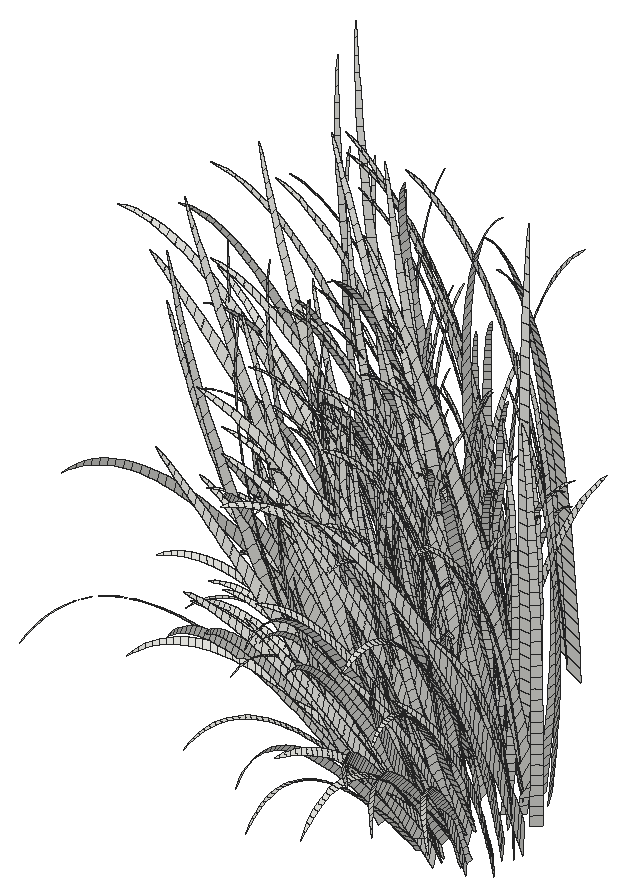
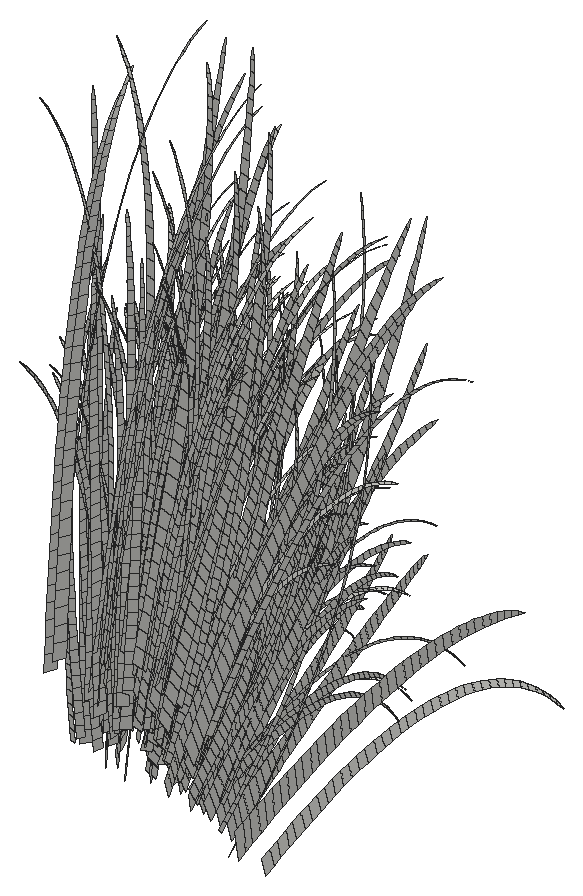
# SketchUp Ruby script. Lengths in inches.
U = 1.inch
M = Sketchup.active_model
def pt(a) = Geom::Point3d.new(a.map { |v| v * U })
def face(e, loops, mat)
  f = e.add_face(loops[0].map { |a| pt(a) })
  loops[1..].each { |l| e.add_face(l.map { |a| pt(a) }).erase! }
  f.material = f.back_material = mat if mat
  f
end
# faces: each face lists its corners as indices into pts; further lists are holes
def faces(e, pts, list, mat = nil) = list.each { |f| face(e, (f[0].is_a?(Array) ? f : [f]).map { |l| l.map { |i| pts[i] } }, mat) }
# xy, xz, yz: faces in a plane at the given z, y or x. An outline is a flat list of corners, or four numbers for a rectangle; further outlines are holes
def ring(l) = l.size == 4 ? [[l[0], l[1]], [l[2], l[1]], [l[2], l[3]], [l[0], l[3]]] : l.each_slice(2).to_a
def flat(e, list, mat, &to3) = list.each { |f| face(e, (f[0].is_a?(Array) ? f : [f]).map { |l| ring(l).map { |u, v| to3.(u, v) } }, mat) }
def xy(e, z, list, mat = nil) = flat(e, list, mat) { |x, y| [x, y, z] }
def xz(e, y, list, mat = nil) = flat(e, list, mat) { |x, z| [x, y, z] }
def yz(e, x, list, mat = nil) = flat(e, list, mat) { |y, z| [x, y, z] }
def lines(e, pts, list) = list.each { |a, b| e.add_line(pt(pts[a]), pt(pts[b])) }
# prism: a flat outline (further loops are holes) pulled along v
def prism(e, loops, v, mat = nil)
  f = face(e, loops, mat); d = Geom::Vector3d.new(v.map { |x| x * U })
  f.pushpull(f.normal.samedirection?(d) ? d.length : -d.length)
end
def box(e, o, s, mat = nil) = prism(e, [[o, [o[0] + s[0], o[1], o[2]], [o[0] + s[0], o[1] + s[1], o[2]], [o[0], o[1] + s[1], o[2]]]], [0, 0, s[2]], mat)
def at(x, y, z, deg = 0) = Geom::Transformation.translation(pt([x, y, z])) * Geom::Transformation.rotation(ORIGIN, Z_AXIS, deg.degrees)
def axes(o, x, y, z) = Geom::Transformation.new([*x, 0, *y, 0, *z, 0, *pt(o).to_a, 1])
def part(name) = M.definitions.add(name)
# library, detail: a bought-in or finely detailed component or shape, given as its bounding box
def library(name, o, s) = part(name).tap { |d| box(d.entities, o, s) }
def detail(e, o, s) = box(e.add_group.entities, o, s)
def put(e, d, t, mat = nil) = e.add_instance(d, t).tap { |i| i.material = mat if mat }
def group(e, t, mat = nil) = e.add_group.tap { |g| g.transformation = t; g.material = mat if mat }.entities
root = M.entities
c1 = part("fur_instance\#8")
p = [[-0.25,1.49,0.03],[0.25,-1.49,-0.03],[0.44,-1.47,1.51],[-0.05,1.47,1.57],[0.65,-1.44,3.05],[0.16,1.45,3.11],
  [0.86,-1.42,4.59],[0.38,1.44,4.65],[1.1,-1.39,6.13],[0.62,1.43,6.18],[1.34,-1.35,7.66],[0.875,1.42,7.72],
  [1.6,-1.32,9.19],[1.14,1.41,9.25],[1.88,-1.28,10.72],[1.43,1.41,10.78],[2.18,-1.24,12.25],[1.73,1.41,12.3],
  [2.49,-1.19,13.77],[2.05,1.41,13.82],[2.83,-1.15,15.29],[2.4,1.41,15.34],[3.18,-1.09,16.8],[2.76,1.42,16.85],
  [3.56,-1.03,18.31],[3.14,1.43,18.35],[3.96,-0.97,19.81],[3.55,1.44,19.85],[4.38,-0.91,21.3],[3.99,1.46,21.35],
  [4.84,-0.83,22.78],[4.45,1.48,22.83],[5.32,-0.76,24.26],[4.93,1.51,24.31],[5.82,-0.67,25.73],[5.45,1.54,25.77],
  [6.36,-0.59,27.18],[6,1.57,27.23],[6.93,-0.49,28.625],[6.58,1.61,28.67],[7.54,-0.39,30.05],[7.19,1.66,30.1],
  [8.18,-0.28,31.47],[7.84,1.71,31.51],[8.85,-0.16,32.86],[8.53,1.77,32.9],[9.57,-0.04,34.24],[9.25,1.83,34.27],
  [10.32,0.09,35.59],[10.02,1.9,35.625],[11.12,0.23,36.92],[10.82,1.97,36.95],[11.95,0.38,38.22],[11.67,2.06,38.25],
  [12.84,0.54,39.49],[12.57,2.14,39.52],[13.76,0.71,40.73],[13.51,2.24,40.76],[14.73,0.89,41.93],[14.49,2.34,41.95],
  [15.75,1.08,43.09],[15.52,2.45,43.11],[16.82,1.28,44.2],[16.6,2.5625,44.23],[17.93,1.5,45.27],[17.73,2.68,45.29],
  [19.08,1.73,46.28],[18.9,2.81,46.3],[20.29,1.97,47.24],[20.125,2.93,47.26],[21.53,2.22,48.13],[21.39,3.0625,48.15],
  [22.82,2.5,48.96],[22.7,3.1875,48.98],[24.14,2.8125,49.72],[24.06,3.3,49.73],[25.48,3.27,50.41]]
faces(c1.entities,p,[[0,1,2,3],[3,2,4,5],[5,4,6,7],[7,6,8,9],[9,8,10,11],[11,10,12,13],[13,12,14,15],[15,14,16,17],
  [17,16,18,19],[19,18,20,21],[21,20,22,23],[23,22,24,25],[25,24,26,27],[27,26,28,29],[29,28,30,31],[31,30,32,33],
  [33,32,34,35],[35,34,36,37],[37,36,38,39],[39,38,40,41],[41,40,42,43],[43,42,44,45],[45,44,46,47],[47,46,48,49],
  [49,48,50,51],[51,50,52,53],[53,52,54,55],[55,54,56,57],[57,56,58,59],[59,58,60,61],[61,60,62,63],[63,62,64,65],
  [65,64,66,67],[67,66,68,69],[69,68,70,71],[71,70,72,73],[73,72,74,75],[75,74,76]])
put(root,c1,axes([41.78,68.76,4.29],[-0.02161,-0.16628,-0.28389],[0.16425,-0.14433,0.32408],[-0.18224,-0.08282,0.344]))
put(root,c1,axes([41.84,66.78,2.31],[-0.07933,-0.07892,-0.44402],[0.19255,-0.17562,0.06989],[-0.14788,-0.14983,0.35337]))
put(root,c1,axes([44.52,67.33,8.31],[-0.23554,0.05296,-0.19778],[0.0198,-0.2043,-0.19606],[-0.09324,-0.11985,0.49597]))
put(root,c1,axes([44.3125,68.95,8.09],[-0.04128,-0.19919,-0.10991],[0.2038,-0.09544,0.23105],[-0.11682,-0.05581,0.46862]))
put(root,c1,axes([43.49,67.08,2.54],[0.13283,-0.0342,0.36955],[-0.05695,0.18902,0.06859],[-0.15898,-0.07225,0.3001]))
put(root,c1,axes([46.45,64.83,3.05],[-0.12873,0.10197,-0.18861],[-0.01018,-0.10343,-0.24101],[-0.11719,-0.08155,0.24232]))
put(root,c1,axes([45.73,68.05,7.22],[-0.08516,-0.14739,-0.15062],[0.16457,-0.13044,0.17116],[-0.1041,-0.04973,0.41758]))
put(root,c1,axes([46.54,64.22,3.46],[-0.15935,0.03269,-0.28558],[0.09029,-0.13292,-0.22683],[-0.09601,-0.14239,0.28508]))
put(root,c1,axes([46.54,64.65,2.75],[-0.14081,0.09765,-0.1356],[-0.01218,-0.08683,-0.27326],[-0.10036,-0.10168,0.23982]))
put(root,c1,axes([46.6875,66.09,7.04],[-0.18347,0.1171,-0.07334],[-0.07461,-0.13251,-0.22152],[-0.07812,-0.10043,0.41558]))
put(root,c1,axes([46.57,64.51,3.25],[-0.15082,0.11254,-0.07354],[-0.05779,-0.09193,-0.25822],[-0.08893,-0.09949,0.31347]))
put(root,c1,axes([46.55,66.52,6.48],[-0.149,-0.04647,-0.21352],[0.09287,-0.17245,0.02054],[-0.09229,-0.06322,0.38876]))
put(root,c1,axes([46.07,64.27,3.58],[-0.09966,0.12678,0.30336],[-0.19172,0.0268,-0.26785],[-0.07616,-0.17634,0.31506]))
put(root,c1,axes([45.32,66.42,3.76],[0.05365,-0.16969,-0.03778],[0.13986,-0.00916,0.27148],[-0.1167,-0.06341,0.32492]))
put(root,c1,axes([46.77,64.77,3.42],[-0.10552,0.13111,0.03774],[-0.1075,-0.03434,-0.24755],[-0.08294,-0.09279,0.29236]))
put(root,c1,axes([47.33,64.85,6.95],[-0.23362,0.09843,0.07428],[-0.08627,-0.11761,-0.36241],[-0.04076,-0.18596,0.42692]))
put(root,c1,axes([46.52,65.09,3.13],[-0.05906,0.14196,0.06951],[-0.12604,0.00717,-0.23329],[-0.09379,-0.07416,0.28621]))
put(root,c1,axes([45.22,65.05,2.3],[0.08197,-0.14846,-0.17255],[0.1435,-0.03613,0.3122],[-0.11735,-0.1189,0.28043]))
put(root,c1,axes([47.35,67.41,9.96],[-0.2227,-0.02851,-0.13015],[0.07795,-0.20389,-0.10631],[-0.04666,-0.10194,0.51151]))
put(root,c1,axes([46.74,65.87,3.48],[-0.05395,-0.10392,-0.15053],[0.10796,-0.10426,0.17042],[-0.10255,-0.03484,0.272]))
put(root,c1,axes([47.33,64.13,4.18],[-0.17727,0.00029,-0.20455],[0.08516,-0.1353,-0.21935],[-0.05731,-0.14134,0.34686]))
put(root,c1,axes([47.08,64.61,4.05],[-0.10062,-0.049,-0.26041],[0.12035,-0.13237,-0.01381],[-0.08638,-0.09663,0.30447]))
put(root,c1,axes([47.39,66.22,4.66],[-0.12457,-0.03797,-0.15408],[0.05979,-0.14532,0.07008],[-0.07901,-0.02356,0.31353]))
put(root,c1,axes([47.03,64.01,4.63],[-0.15374,0.14658,0.25603],[-0.19784,-0.04817,-0.27014],[-0.04101,-0.18709,0.42951]))
put(root,c1,axes([45.42,65.41,2.3],[0.13307,-0.06357,0.27984],[-0.03809,0.14212,0.17121],[-0.12562,-0.08741,0.25976]))
put(root,c1,axes([47.3,64.3,2.92],[-0.0986,0.1202,0.03133],[-0.09749,-0.03341,-0.22837],[-0.07635,-0.08541,0.26912]))
put(root,c1,axes([47.09,64.0625,2.52],[-0.08725,-0.02366,-0.29756],[0.12591,-0.11202,-0.06714],[-0.0803,-0.1191,0.23844]))
put(root,c1,axes([47.62,64.14,3.49],[-0.15103,0.03829,-0.1475],[0.02836,-0.11444,-0.19385],[-0.06472,-0.10394,0.28282]))
put(root,c1,axes([44.92,65.9,4.11],[0.17403,-0.06722,0.24815],[-0.01797,0.16553,0.179],[-0.11789,-0.09322,0.35975]))
put(root,c1,axes([46.59,63.5625,2.5],[-0.07738,0.12181,0.42116],[-0.24475,0.02807,-0.19007],[-0.04925,-0.2161,0.35893]))
put(root,c1,axes([47.8,63.58,3.5],[-0.19758,0.0885,0.1271],[-0.09447,-0.05952,-0.37318],[-0.04202,-0.18438,0.30623]))
put(root,c1,axes([46.29,65.45,3.97],[0.04667,0.10587,0.22641],[-0.14224,0.11026,-0.13144],[-0.10087,-0.07976,0.30781]))
put(root,c1,axes([47.18,65,6.72],[-0.12023,0.16893,0.15811],[-0.19192,-0.04724,-0.20175],[-0.05017,-0.13536,0.45159]))
put(root,c1,axes([47.44,64.82,5.0625],[-0.1513,-0.02821,-0.17374],[0.08683,-0.1419,-0.10144],[-0.05423,-0.09755,0.35603]))
put(root,c1,axes([47.56,64.62,3.98],[-0.07947,0.12548,0.07397],[-0.11521,-0.01055,-0.22059],[-0.07706,-0.08621,0.27164]))
put(root,c1,axes([47.27,66.85,4.41],[-0.06439,-0.12354,-0.04587],[0.12333,-0.08786,0.16125],[-0.07712,-0.0102,0.31415]))
put(root,c1,axes([46.72,65.11,3.03],[0.02731,-0.14018,-0.06519],[0.12315,-0.02871,0.2214],[-0.09827,-0.0534,0.27359]))
put(root,c1,axes([46.11,64.66,2.43],[0.09631,-0.13966,-0.10726],[0.11682,-0.00954,0.30869],[-0.10751,-0.10893,0.25692]))
put(root,c1,axes([48.04,64.74,5.63],[-0.18173,0.02045,-0.09763],[0.0261,-0.14072,-0.18343],[-0.04068,-0.10974,0.36609]))
put(root,c1,axes([46.52,65.89,3.82],[0.06905,-0.15041,0.07394],[0.1069,0.0384,0.22809],[-0.10814,-0.03674,0.28683]))
put(root,c1,axes([46.49,66.28,5.39],[0.02994,-0.16585,-0.05499],[0.16129,-0.01842,0.19273],[-0.08623,-0.05907,0.36324]))
put(root,c1,axes([48.125,63.5,3.07],[-0.18497,0.04944,-0.02341],[-0.00878,-0.07542,-0.33252],[-0.03553,-0.1559,0.25894]))
put(root,c1,axes([47.84,65.75,5.99],[-0.14413,-0.05167,-0.11933],[0.08701,-0.14734,-0.01287],[-0.04763,-0.0596,0.37283]))
put(root,c1,axes([47.56,63.85,2.69],[-0.04193,0.09854,0.23039],[-0.14173,0.04993,-0.18317],[-0.07748,-0.11492,0.23007]))
put(root,c1,axes([47.32,66.04,4.73],[-0.02354,-0.13666,-0.06934],[0.13862,-0.06024,0.1585],[-0.07899,-0.03774,0.31687]))
put(root,c1,axes([48.28,63.625,3.125],[-0.15528,0.03655,-0.09389],[0.01601,-0.10098,-0.21878],[-0.04549,-0.11219,0.27533]))
put(root,c1,axes([48.32,64.46,4.68],[-0.15238,0.03287,-0.097],[0.00948,-0.12228,-0.14695],[-0.04746,-0.08538,0.3116]))
put(root,c1,axes([47.56,65.7,5.13],[-0.02967,-0.13006,-0.11002],[0.14258,-0.07093,0.13984],[-0.07655,-0.05244,0.32247]))
put(root,c1,axes([46.44,65.01,3.49],[0.10962,-0.14134,0.02858],[0.09848,0.05163,0.25611],[-0.09929,-0.07851,0.30299]))
put(root,c1,axes([47.93,65.02,5.84],[-0.07622,0.14548,0.11566],[-0.15943,-0.01772,-0.1678],[-0.05494,-0.09882,0.36066]))
put(root,c1,axes([48.65,65.69,8.6],[-0.23536,0.00031,-0.04255],[0.03502,-0.16941,-0.26023],[-0.00865,-0.15175,0.46324]))
put(root,c1,axes([47.03,63.92,2.59],[0.07176,0.04443,0.32956],[-0.1495,0.11571,0.02095],[-0.08693,-0.12893,0.25813]))
put(root,c1,axes([48.18,67.92,9.34],[-0.16552,-0.11118,-0.05649],[0.14207,-0.16762,-0.00154],[-0.02412,-0.05905,0.48802]))
put(root,c1,axes([48.14,63.68,3.9375],[-0.1192,0.12425,0.22535],[-0.17166,-0.03356,-0.21354],[-0.0342,-0.15606,0.35826]))
put(root,c1,axes([47.85,65.45,5.16],[-0.02927,-0.12714,-0.10789],[0.13946,-0.06963,0.13664],[-0.0749,-0.05131,0.31553]))
put(root,c1,axes([46.1,64.84,4.72],[0.13498,-0.15634,-0.12045],[0.15269,0.03421,0.29976],[-0.08583,-0.13785,0.37509]))
put(root,c1,axes([47.34,66.07,8.47],[-0.00008,0.17023,0.2439],[-0.22913,0.05018,-0.08813],[-0.05076,-0.13695,0.4569]))
put(root,c1,axes([46.17,66.21,6.04],[0.15632,-0.13539,0.07566],[0.09629,0.11232,0.20743],[-0.0859,-0.08088,0.3964]))
put(root,c1,axes([46.0625,63.875,2.7],[0.17581,0.00429,0.35889],[-0.15371,0.13999,0.25001],[-0.08231,-0.1906,0.34052]))
put(root,c1,axes([47.25,65.44,6.82],[0.05112,0.14176,0.22694],[-0.19757,0.09246,-0.06236],[-0.06344,-0.11412,0.4165]))
put(root,c1,axes([47.59,65.46,5.51],[0.0229,-0.1484,-0.09458],[0.15576,-0.02704,0.16403],[-0.07366,-0.06935,0.33993]))
put(root,c1,axes([47.875,67.02,8.52],[-0.04613,-0.168,-0.12838],[0.20048,-0.07761,0.07112],[-0.05022,-0.08162,0.45074]))
put(root,c1,axes([47.39,66.9375,7.59],[0.01336,-0.18156,-0.05149],[0.1916,-0.02315,0.12623],[-0.05991,-0.05859,0.42926]))
put(root,c1,axes([46.94,65.12,3.85],[0.13306,-0.03251,0.2141],[-0.03468,0.1366,0.1095],[-0.09265,-0.07326,0.28274]))
put(root,c1,axes([48.44,65.3,7.09],[-0.14651,-0.09517,-0.11625],[0.13838,-0.13795,-0.08263],[-0.01824,-0.0963,0.42995]))
put(root,c1,axes([49.16,66.82,9.55],[-0.22374,-0.02944,-0.01516],[0.05551,-0.18692,-0.16154],[0.00543,-0.11272,0.49003]))
put(root,c1,axes([48.06,63.75,3.63],[-0.00857,-0.10681,-0.26092],[0.17656,-0.05814,0.06779],[-0.05152,-0.12704,0.31177]))
put(root,c1,axes([46.96,64.66,4.28],[0.14194,0.01295,0.23971],[-0.09799,0.13483,0.13149],[-0.07264,-0.11667,0.31745]))
put(root,c1,axes([47.82,64.1875,3.83],[0.04246,-0.11664,-0.17724],[0.14637,-0.02684,0.16417],[-0.06419,-0.10309,0.2805]))
put(root,c1,axes([48.97,66.82,7.8],[-0.13872,-0.10688,-0.05008],[0.13478,-0.14007,-0.01499],[-0.01621,-0.05768,0.43132]))
put(root,c1,axes([48.61,67.18,7.55],[-0.09202,-0.14419,-0.02135],[0.16494,-0.10399,0.03603],[-0.02333,-0.03794,0.42396]))
put(root,c1,axes([47.79,66.01,5.16],[0.09225,-0.12894,0.11038],[0.10291,0.0771,0.12838],[-0.07903,-0.02356,0.31361]))
put(root,c1,axes([47.93,63.42,2.29],[0.04168,-0.09258,-0.28201],[0.16554,-0.04371,0.15063],[-0.06017,-0.13932,0.24891]))
put(root,c1,axes([47.09,64.72,4.5],[0.15549,-0.01208,0.20833],[-0.06905,0.13306,0.17126],[-0.07165,-0.11508,0.31313]))
put(root,c1,axes([49.47,65.93,7.63],[-0.18618,-0.03996,-0.02577],[0.06509,-0.15689,-0.1364],[0.00464,-0.09644,0.41925]))
put(root,c1,axes([49.48,65.55,6.21],[-0.15853,0.06077,0.01255],[-0.05151,-0.13731,-0.04414],[-0.00488,-0.05314,0.37046]))
put(root,c1,axes([49.9,64.09,5.82],[-0.25079,-0.01126,0.01167],[0.02691,-0.14432,-0.37072],[0.02191,-0.19373,0.42855]))
put(root,c1,axes([49.36,63.75,4.3125],[-0.15193,-0.01941,-0.09588],[0.0644,-0.09304,-0.22233],[-0.00624,-0.12588,0.27933]))
put(root,c1,axes([49.66,62.98,2.04],[-0.16406,0.03446,0.0684],[-0.03839,-0.06194,-0.29017],[-0.00638,-0.14462,0.2315]))
put(root,c1,axes([46.76,63.98,2.88],[0.18766,-0.05407,0.15304],[-0.0375,0.10124,0.3241],[-0.06745,-0.15619,0.27904]))
put(root,c1,axes([48.46,65.78,9],[-0.04308,0.17847,0.273],[-0.24701,-0.00413,-0.05166],[-0.00912,-0.15991,0.48813]))
put(root,c1,axes([47.83,64.11,4.75],[0.03417,-0.12525,-0.29157],[0.20378,-0.0224,0.09589],[-0.03382,-0.15429,0.3542]))
put(root,c1,axes([48.12,64.54,6.09],[0.00591,-0.15376,-0.2335],[0.21361,-0.03099,0.04882],[-0.02765,-0.13326,0.41924]))
put(root,c1,axes([48.92,64.44,6.04],[-0.06192,0.14505,0.21697],[-0.19671,-0.02273,-0.07174],[-0.0075,-0.13152,0.40147]))
put(root,c1,axes([50.16,63.75,4.72],[-0.22603,-0.01056,0.00948],[0.02497,-0.13008,-0.33426],[0.01976,-0.17466,0.38636]))
put(root,c1,axes([48.68,65.36,7.52],[0.0038,0.14954,0.23139],[-0.20994,0.03733,-0.03743],[-0.02717,-0.13094,0.41195]))
put(root,c1,axes([48.78,65.625,5.72],[-0.04654,-0.13259,-0.03011],[0.14978,-0.05997,0.02545],[-0.01873,-0.03986,0.3514]))
put(root,c1,axes([48.82,63.08,2.03],[-0.02123,-0.06781,-0.31584],[0.17417,-0.05199,-0.00113],[-0.03366,-0.14772,0.24534]))
put(root,c1,axes([49.7,64.51,6.78],[-0.18897,-0.07724,-0.16578],[0.14014,-0.11074,-0.30364],[0.02044,-0.18069,0.39971]))
put(root,c1,axes([48.85,65.26,7.03],[-0.0211,0.16438,0.13367],[-0.19675,0.00758,-0.04177],[-0.01791,-0.09455,0.42215]))
put(root,c1,axes([49.51,66.02,7.33],[-0.1296,-0.11177,-0.03307],[0.13714,-0.12794,-0.0397],[-0.00189,-0.06022,0.41924]))
put(root,c1,axes([48.35,63.68,3.39],[0.0606,-0.10906,-0.18612],[0.14677,-0.00638,0.15494],[-0.04628,-0.11412,0.28007]))
put(root,c1,axes([49.9375,65.31,7.9375],[-0.15736,0.12863,0.21317],[-0.17096,-0.10355,-0.14422],[0.01307,-0.14881,0.45294]))
put(root,c1,axes([49.875,64.49,5.75],[-0.16225,-0.04777,-0.05886],[0.07812,-0.11873,-0.19059],[0.01013,-0.11533,0.35104]))
put(root,c1,axes([49.71,65.42,6.76],[-0.13495,-0.09194,-0.07228],[0.12419,-0.11921,-0.10694],[0.00432,-0.08968,0.38985]))
put(root,c1,axes([48.85,66.05,7.53],[-0.00432,-0.15952,-0.128],[0.19173,-0.03266,0.04648],[-0.02798,-0.08806,0.41192]))
put(root,c1,axes([48.375,63.94,4.2],[0.10535,0.0488,0.23666],[-0.12967,0.10407,0.09442],[-0.04869,-0.12008,0.29468]))
put(root,c1,axes([48.85,66.96,6.97],[-0.00822,-0.16722,0.01164],[0.17876,-0.02595,0.03382],[-0.01925,-0.0303,0.40131]))
put(root,c1,axes([49.99,64.4,5.2],[-0.14242,0.06423,0.07833],[-0.06984,-0.11466,-0.07925],[0.01251,-0.07634,0.33832]))
put(root,c1,axes([50.04,64.98,6.57],[-0.1422,0.11091,0.11586],[-0.12628,-0.11191,-0.06649],[0.015,-0.09153,0.40561]))
put(root,c1,axes([50.3,67.46,8.9],[-0.17633,-0.09809,0.01724],[0.1199,-0.16919,-0.04915],[0.01352,-0.05835,0.47546]))
put(root,c1,axes([50.07,63.61,4.08],[-0.13701,0.06738,0.19305],[-0.11347,-0.07671,-0.17654],[0.01546,-0.13663,0.30225]))
put(root,c1,axes([50.05,65.19,6.03],[-0.14765,0.06695,0.09599],[-0.07527,-0.12279,-0.06548],[0.02169,-0.07701,0.35566]))
put(root,c1,axes([50.42,67.52,9.97],[-0.22223,-0.05187,0.06437],[0.06185,-0.19269,-0.14793],[0.04097,-0.1013,0.49904]))
put(root,c1,axes([48.05,66.37,6.47],[0.1666,-0.05285,0.10887],[0.0248,0.15525,0.04679],[-0.05548,-0.04238,0.37888]))
put(root,c1,axes([49.94,63.07,2.46],[-0.13424,-0.03889,-0.12787],[0.08866,-0.05443,-0.25596],[0.01839,-0.13945,0.22254]))
put(root,c1,axes([49.15,64.55,5.62],[0.0286,0.11518,0.18982],[-0.16763,0.04809,-0.0018],[-0.022,-0.10604,0.33361]))
put(root,c1,axes([48.57,64.7,5.24],[0.09089,0.09523,0.11248],[-0.12952,0.09997,0.00707],[-0.03129,-0.06837,0.34303]))
put(root,c1,axes([49.31,64.97,5.66],[0.0055,0.12915,0.11043],[-0.15799,0.02454,-0.01796],[-0.01431,-0.07554,0.33727]))
put(root,c1,axes([47.59,66.85,8.375],[0.2061,-0.01344,0.1131],[-0.02793,0.18662,0.09605],[-0.05077,-0.08252,0.4557]))
put(root,c1,axes([49.52,63.37,3.39],[-0.02267,0.09523,0.24051],[-0.16406,0.00552,-0.03477],[-0.00627,-0.12634,0.28034]))
put(root,c1,axes([48.4,65.7,6.31],[0.13539,0.06511,0.11886],[-0.10233,0.13809,0.02305],[-0.04143,-0.06734,0.37184]))
put(root,c1,axes([50.24,66.6,7.25],[-0.12883,-0.11449,0.01319],[0.1336,-0.12723,-0.04151],[0.01291,-0.04776,0.41418]))
put(root,c1,axes([48.67,66.85,10.16],[0.02992,-0.20268,-0.17218],[0.24479,0.00013,0.02509],[-0.00825,-0.12029,0.52424]))
put(root,c1,axes([50.33,68.1,10.78],[-0.1863,-0.12854,0.00057],[0.15019,-0.16226,-0.16735],[0.0425,-0.10509,0.5177]))
put(root,c1,axes([49.84,66.31,6.62],[-0.07961,-0.13689,0.01423],[0.15313,-0.0843,-0.034],[0.01219,-0.0383,0.38556]))
put(root,c1,axes([49.83,66.73,7.03],[-0.07772,-0.14595,0.01956],[0.16231,-0.0838,-0.0308],[0.01178,-0.03674,0.40206]))
put(root,c1,axes([49.89,66.22,6.24],[-0.07124,-0.13476,0.02236],[0.14958,-0.07747,-0.02272],[0.00941,-0.03103,0.37011]))
put(root,c1,axes([49.61,63.66,4.18],[0.01737,0.09262,0.24572],[-0.16736,0.02852,0.02395],[-0.00637,-0.12835,0.28481]))
put(root,c1,axes([47.98,67.91,10.81],[0.18706,-0.15692,-0.05371],[0.1539,0.13296,0.16341],[-0.03534,-0.11123,0.5203]))
put(root,c1,axes([48.73,64.9375,5.4375],[0.13738,0.0414,0.0972],[-0.07592,0.13055,0.05523],[-0.03104,-0.06782,0.34028]))
put(root,c1,axes([50.12,64.96,6.6],[-0.07914,0.12591,0.21103],[-0.17333,-0.05924,-0.02394],[0.02804,-0.12033,0.37519]))
put(root,c1,axes([50.22,64.61,5.97],[-0.10701,-0.11213,-0.12442],[0.15233,-0.07687,-0.16606],[0.02739,-0.11756,0.36656]))
put(root,c1,axes([50.87,64.56,5.34],[-0.16995,0.00239,0.1052],[-0.0155,-0.13112,-0.16118],[0.04006,-0.1041,0.34197]))
put(root,c1,axes([48.71,63.27,2.98],[0.11054,0.06076,0.32124],[-0.18174,0.06569,0.1961],[-0.00805,-0.18258,0.29226]))
put(root,c1,axes([49.21,66.46,8.56],[0.04164,-0.17352,-0.14577],[0.20763,0.01338,0.03275],[-0.00709,-0.10329,0.45016]))
put(root,c1,axes([49.16,63.36,3.25],[0.07036,0.07691,0.22077],[-0.15002,0.05652,0.10186],[-0.00627,-0.1264,0.28049]))
put(root,c1,axes([48.73,65.46,6.65],[0.15043,0.06237,0.10618],[-0.10193,0.14112,0.07332],[-0.02651,-0.08344,0.39031]))
put(root,c1,axes([48.8125,64.57,5.39],[0.1599,-0.01285,0.09328],[-0.0299,0.12534,0.15874],[-0.03604,-0.09723,0.32437]))
put(root,c1,axes([51.14,63.47,3.49],[-0.19796,-0.00213,0.19119],[-0.0584,-0.09827,-0.32515],[0.05556,-0.17894,0.29438]))
put(root,c1,axes([49.65,64.5,5.97],[-0.00485,-0.13574,-0.20923],[0.19174,-0.01245,-0.03687],[0.01079,-0.12284,0.3739]))
put(root,c1,axes([48.62,64.14,4.84],[0.16477,0.01322,0.09468],[-0.05646,0.12716,0.16983],[-0.02254,-0.10862,0.34171]))
put(root,c1,axes([51.28,66.57,7.14],[-0.18521,-0.02955,0.11381],[0.03239,-0.17376,-0.06029],[0.05035,-0.05919,0.41626]))
put(root,c1,axes([51.02,64.2,4.41],[-0.14955,-0.02951,0.08847],[0.01953,-0.12021,-0.14832],[0.04773,-0.08667,0.30915]))
put(root,c1,axes([49,63.6,3.82],[0.16669,-0.01734,0.08094],[-0.02966,0.10281,0.23812],[-0.02771,-0.12642,0.29024]))
put(root,c1,axes([49.2,63.39,3.51],[0.12347,0.06755,0.21237],[-0.14396,0.08585,0.17984],[-0.00718,-0.14468,0.32104]))
put(root,c1,axes([51.18,65.25,7.42],[-0.16708,-0.12567,-0.06302],[0.15179,-0.11958,-0.24667],[0.05298,-0.1377,0.45233]))
put(root,c1,axes([49.3,67.21,6.92],[0.10751,-0.14401,0.02773],[0.14274,0.0886,-0.01156],[-0.00773,-0.0245,0.39927]))
put(root,c1,axes([50.39,63.22,2.98],[-0.04322,-0.08103,-0.33227],[0.19342,-0.01502,-0.11763],[0.02265,-0.17179,0.27415]))
put(root,c1,axes([50.66,66.19,5.78],[-0.08777,-0.12311,0.07978],[0.13105,-0.09185,-0.0647],[0.04014,-0.02395,0.34954]))
put(root,c1,axes([51.1875,64.67,6.28],[-0.14817,-0.12463,-0.07303],[0.15181,-0.10509,-0.22784],[0.04979,-0.1294,0.42509]))
put(root,c1,axes([49.47,64.26,5.16],[0.12885,0.05972,0.11755],[-0.10424,0.10176,0.1411],[-0.00603,-0.1057,0.32265]))
put(root,c1,axes([51.13,63.19,2.1],[-0.14554,-0.04613,0.08103],[0.01279,-0.07284,-0.26823],[0.06295,-0.12513,0.21981]))
put(root,c1,axes([51.38,64.25,5.13],[-0.14966,0.06135,0.2769],[-0.12806,-0.11932,-0.12286],[0.06613,-0.14624,0.35295]))
put(root,c1,axes([51.13,63.18,2.18],[-0.08929,0.05587,0.30832],[-0.15159,-0.06244,-0.09121],[0.04736,-0.15254,0.25094]))
put(root,c1,axes([49.3,65.71,6.21],[0.16373,-0.03857,0.00921],[0.02397,0.14494,0.04432],[-0.01107,-0.05099,0.36849]))
put(root,c1,axes([50.56,65.56,5.93],[-0.04201,-0.14205,-0.02716],[0.15521,-0.03808,-0.10788],[0.03986,-0.0584,0.35377]))
put(root,c1,axes([49.49,63.04,2.3],[0.15269,-0.07243,-0.24019],[0.13551,0.04613,0.26977],[-0.00773,-0.17522,0.28049]))
put(root,c1,axes([49.54,64.98,5.84],[0.14874,-0.07113,-0.04632],[0.06911,0.1145,0.10604],[-0.00549,-0.08,0.34865]))
put(root,c1,axes([51.38,65.57,5.34],[-0.14662,-0.03521,0.15792],[0.02351,-0.14317,-0.07806],[0.07228,-0.05609,0.32502]))
put(root,c1,axes([49.42,66.05,6.65],[0.16142,-0.07143,-0.01571],[0.0631,0.13884,0.04506],[-0.00507,-0.05525,0.3852]))
put(root,c1,axes([49.45,67.26,8.02],[0.12208,-0.15013,-0.02869],[0.15272,0.10311,-0.03034],[0.01381,-0.04339,0.43679]))
put(root,c1,axes([51.625,64.5625,6.29],[-0.10088,0.13062,0.3695],[-0.228,-0.07812,-0.04804],[0.0527,-0.18996,0.43195]))
put(root,c1,axes([49.73,63,2.23],[0.1143,0.07759,0.29786],[-0.18253,0.04472,0.24081],[0.02462,-0.18668,0.29791]))
put(root,c1,axes([49.9,65.15,6.76],[0.10618,-0.13596,-0.12929],[0.15853,0.08066,0.0353],[0.01505,-0.09183,0.40695]))
put(root,c1,axes([51.01,64.25,5.47],[-0.04153,-0.12718,-0.27595],[0.20481,-0.00989,-0.14624],[0.04417,-0.15922,0.36205]))
put(root,c1,axes([49.59,63.21,3.07],[0.19045,-0.03751,-0.06848],[0.03839,0.07261,0.33686],[-0.00736,-0.16676,0.26694]))
put(root,c1,axes([50.17,65.09,6.18],[0.0987,0.11897,0.05521],[-0.14378,0.08662,0.10909],[0.02282,-0.08103,0.37425]))
put(root,c1,axes([50.14,66.72,6.34],[0.11708,-0.12342,-0.00631],[0.12225,0.10057,-0.03033],[0.0076,-0.02912,0.37804]))
put(root,c1,axes([50.12,63.2,2.97],[0.10158,-0.06914,-0.32205],[0.1701,0.0448,0.14301],[0.02265,-0.17174,0.27406]))
put(root,c1,axes([51.04,63.58,3.59],[0.00165,-0.10984,-0.26082],[0.18149,0.01453,-0.07449],[0.03836,-0.13829,0.31445]))
put(root,c1,axes([52.35,65.85,7.3],[-0.1604,-0.13739,-0.02167],[0.15059,-0.11716,-0.25101],[0.06963,-0.12643,0.45099]))
put(root,c1,axes([53.03,64.98,5.97],[-0.21667,0.03837,0.29524],[-0.10928,-0.16078,-0.2283],[0.08148,-0.18018,0.43484]))
put(root,c1,axes([50.07,63.9,4.52],[0.15315,-0.04031,-0.07636],[0.04669,0.1064,0.16007],[0.009,-0.10254,0.31211]))
put(root,c1,axes([52.5,64.41,4.1875],[-0.18644,-0.03104,0.19118],[-0.0143,-0.14214,-0.22961],[0.08573,-0.13206,0.3504]))
put(root,c1,axes([50.83,65.08,5.99],[0.0438,-0.14683,-0.11127],[0.16937,0.03664,-0.05087],[0.03107,-0.07683,0.37846]))
put(root,c1,axes([52.51,67.99,10.49],[-0.20857,-0.13075,0.08955],[0.12369,-0.16885,-0.26752],[0.09431,-0.12712,0.50956]))
put(root,c1,axes([50.35,65.82,5.9],[0.13914,-0.08385,-0.03496],[0.08075,0.12335,-0.00894],[0.01158,-0.03859,0.35924]))
put(root,c1,axes([52.07,63.78,2.13],[-0.12758,-0.07753,0.0557],[0.04435,-0.06394,-0.27127],[0.08127,-0.11212,0.2187]))
put(root,c1,axes([52.35,64.0625,2.84],[-0.14977,-0.06071,0.14936],[0.00439,-0.0935,-0.26844],[0.09015,-0.12438,0.2426]))
put(root,c1,axes([51.72,64.36,3.93],[-0.08522,-0.11751,-0.02593],[0.11177,-0.04315,-0.23298],[0.08081,-0.09116,0.27707]))
put(root,c1,axes([50.51,63.84,4.31],[0.12624,-0.07118,-0.14847],[0.09892,0.09301,0.09957],[0.0236,-0.10128,0.3158]))
put(root,c1,axes([50.33,65.81,6.67],[0.11075,-0.11944,-0.11937],[0.13443,0.0987,-0.0216],[0.03784,-0.07056,0.38011]))
put(root,c1,axes([49.5625,66.85,10.4375],[0.24074,-0.08114,-0.0797],[0.07823,0.19128,0.15934],[0.00596,-0.12377,0.53808]))
put(root,c1,axes([53.36,64.16,3.67],[-0.23798,-0.07441,0.13592],[0.01899,-0.11962,-0.43721],[0.10286,-0.20447,0.35918]))
put(root,c1,axes([51.99,64.73,4.11],[-0.09743,0.06774,0.23139],[-0.09599,-0.11967,0.05358],[0.09249,-0.07723,0.28321]))
put(root,c1,axes([51.64,64.89,5.91],[-0.02184,-0.15888,-0.15748],[0.19236,-0.00034,-0.15603],[0.06127,-0.11125,0.39683]))
put(root,c1,axes([50.43,65.52,5.86],[0.15222,0.03642,-0.07852],[-0.03946,0.13914,0.07531],[0.03898,-0.05711,0.34597]))
put(root,c1,axes([52.34,65.35,3.95],[-0.11286,0.04976,0.22948],[-0.06771,-0.13658,0.05175],[0.0986,-0.05954,0.28318]))
put(root,c1,axes([51.05,66.85,6.82],[0.07494,-0.15978,-0.03962],[0.16264,0.06715,-0.11216],[0.04856,-0.037,0.39794]))
put(root,c1,axes([52.39,65.16,5.16],[-0.12334,-0.12969,0.01714],[0.11431,-0.07492,-0.27994],[0.09668,-0.10907,0.33149]))
put(root,c1,axes([50.88,63.32,2.99],[0.09702,-0.05494,-0.31246],[0.152,0.06601,0.10474],[0.04854,-0.15634,0.25719]))
put(root,c1,axes([52.02,68.49,10.01],[-0.02329,-0.21903,-0.03429],[0.23378,-0.02287,-0.15724],[0.06291,-0.07396,0.52011]))
put(root,c1,axes([50.81,66.1,5.52],[0.13682,-0.07692,-0.07129],[0.07213,0.1295,-0.07116],[0.03936,-0.02349,0.34277]))
put(root,c1,axes([50.36,63.61,4.39],[0.22137,0.04305,0.07377],[-0.08148,0.12835,0.33894],[0.02049,-0.18118,0.40078]))
put(root,c1,axes([50.76,63.89,4.47],[0.16263,0.05278,0.0273],[-0.0671,0.09353,0.2615],[0.03718,-0.13404,0.3048]))
put(root,c1,axes([50.64,66.0625,6.28],[0.1463,-0.07615,-0.10409],[0.07711,0.13848,-0.04067],[0.04559,-0.04329,0.3674]))
put(root,c1,axes([52.79,66.03,4.71],[-0.14023,0.01888,0.26296],[-0.04453,-0.1614,-0.00292],[0.11023,-0.06656,0.31656]))
put(root,c1,axes([52.66,64.38,2.89],[-0.13012,-0.10057,0.10963],[0.04873,-0.08061,-0.28847],[0.10836,-0.10823,0.24566]))
put(root,c1,axes([51.23,65.97,5.6],[0.10839,-0.11453,-0.08174],[0.11795,0.10157,-0.07097],[0.04416,-0.04194,0.35588]))
put(root,c1,axes([51.03,65.1,7.5],[0.14666,-0.13638,-0.25039],[0.18844,0.10867,0.09026],[0.03514,-0.1508,0.47019]))
put(root,c1,axes([53.0625,66.26,4.54],[-0.14894,-0.04461,0.24591],[0.01234,-0.15892,-0.10432],[0.11196,-0.06761,0.32156]))
put(root,c1,axes([52.61,68.4,9.23],[-0.02212,-0.21398,-0.03391],[0.22838,-0.02174,-0.15347],[0.06144,-0.07223,0.50797]))
put(root,c1,axes([50.58,66.9,9.57],[0.23315,0.01342,-0.06471],[-0.02237,0.19719,0.15093],[0.03065,-0.10883,0.50265]))
put(root,c1,axes([51.34,65.17,5.41],[0.10539,0.11766,-0.04264],[-0.11395,0.08648,0.1779],[0.06944,-0.07112,0.33381]))
put(root,c1,axes([53.27,65.09,3.87],[-0.10089,0.09227,0.28247],[-0.13958,-0.12254,0.05217],[0.09902,-0.11171,0.33951]))
put(root,c1,axes([52.67,65.4,6.49],[-0.03936,0.14543,0.30601],[-0.20696,-0.07562,0.14027],[0.09659,-0.14879,0.39477]))
